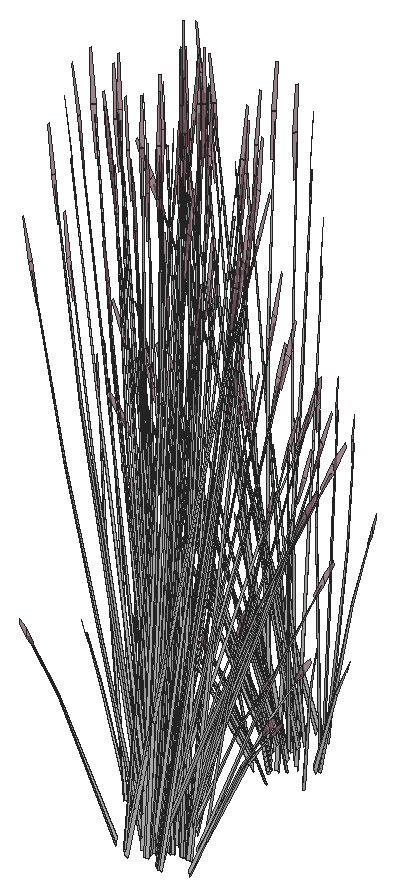
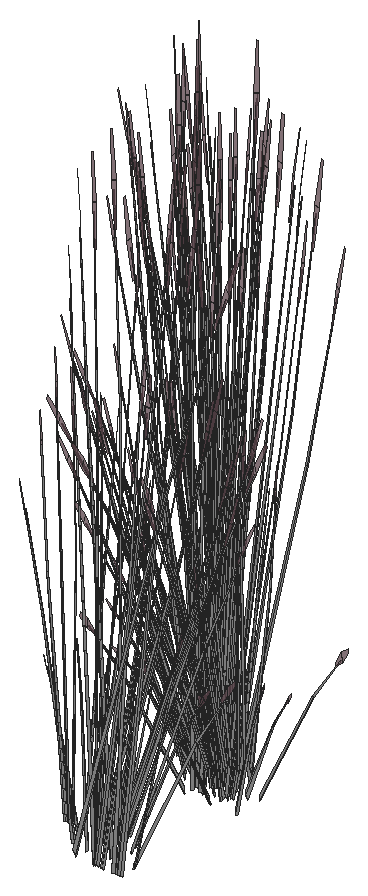
# SketchUp Ruby script. Lengths in inches.
U = 1.inch
M = Sketchup.active_model
def pt(a) = Geom::Point3d.new(a.map { |v| v * U })
def face(e, loops, mat)
  f = e.add_face(loops[0].map { |a| pt(a) })
  loops[1..].each { |l| e.add_face(l.map { |a| pt(a) }).erase! }
  f.material = f.back_material = mat if mat
  f
end
# faces: each face lists its corners as indices into pts; further lists are holes
def faces(e, pts, list, mat = nil) = list.each { |f| face(e, (f[0].is_a?(Array) ? f : [f]).map { |l| l.map { |i| pts[i] } }, mat) }
# xy, xz, yz: faces in a plane at the given z, y or x. An outline is a flat list of corners, or four numbers for a rectangle; further outlines are holes
def ring(l) = l.size == 4 ? [[l[0], l[1]], [l[2], l[1]], [l[2], l[3]], [l[0], l[3]]] : l.each_slice(2).to_a
def flat(e, list, mat, &to3) = list.each { |f| face(e, (f[0].is_a?(Array) ? f : [f]).map { |l| ring(l).map { |u, v| to3.(u, v) } }, mat) }
def xy(e, z, list, mat = nil) = flat(e, list, mat) { |x, y| [x, y, z] }
def xz(e, y, list, mat = nil) = flat(e, list, mat) { |x, z| [x, y, z] }
def yz(e, x, list, mat = nil) = flat(e, list, mat) { |y, z| [x, y, z] }
def lines(e, pts, list) = list.each { |a, b| e.add_line(pt(pts[a]), pt(pts[b])) }
# prism: a flat outline (further loops are holes) pulled along v
def prism(e, loops, v, mat = nil)
  f = face(e, loops, mat); d = Geom::Vector3d.new(v.map { |x| x * U })
  f.pushpull(f.normal.samedirection?(d) ? d.length : -d.length)
end
def box(e, o, s, mat = nil) = prism(e, [[o, [o[0] + s[0], o[1], o[2]], [o[0] + s[0], o[1] + s[1], o[2]], [o[0], o[1] + s[1], o[2]]]], [0, 0, s[2]], mat)
def at(x, y, z, deg = 0) = Geom::Transformation.translation(pt([x, y, z])) * Geom::Transformation.rotation(ORIGIN, Z_AXIS, deg.degrees)
def axes(o, x, y, z) = Geom::Transformation.new([*x, 0, *y, 0, *z, 0, *pt(o).to_a, 1])
def part(name) = M.definitions.add(name)
# library, detail: a bought-in or finely detailed component or shape, given as its bounding box
def library(name, o, s) = part(name).tap { |d| box(d.entities, o, s) }
def detail(e, o, s) = box(e.add_group.entities, o, s)
def put(e, d, t, mat = nil) = e.add_instance(d, t).tap { |i| i.material = mat if mat }
def group(e, t, mat = nil) = e.add_group.tap { |g| g.transformation = t; g.material = mat if mat }.entities
root = M.entities
M.materials.add("LightPink_Translucent").color = [144, 107, 117]
M.materials["LightPink_Translucent"].alpha = 0.75
M.materials.add("[_0053_Ivory_]").color = [200, 200, 200]
c1 = part("blade")
p = [[2.15,0.21,22],[0,0.17,0],[0.09,0.45,0],[2.18,0.31,22],[2.29,0.31,22],[0.38,0.45,0],
  [2.48,0.24,33],[2.49,0.24,33],[2.48,0.22,33]]
faces(c1.entities,p,[[0,1,2,3],[4,5,2,3],[6,3,4,7],[8,0,3,6]])
c2 = part("seeds")
p = [[0.3,-0.1,1.38],[-0.01,-0.03,1.59],[-0.01,-0.03,0.03],[0.14,-0.07,-0.07],[0.29,-0.03,3],[0.15,0.01,3.11]]
faces(c2.entities,p,[[0,1,2,3],[1,0,4,5]],"LightPink_Translucent")
c3 = part("blade with seeds")
put(c3.entities,c1,at(0,0,0))
put(c3.entities,c2,axes([2.4,0.25,30.99],[1.5799,-0.05474,1.17369],[-0.12525,1.92788,0.29478],[-0.07173,-0.02425,1.56792]))
put(root,c3,axes([642.95,172.91,128.71],[-0.63179,-0.1031,-0.62353],[0.13332,-0.63596,-0.16365],[-0.18854,-0.07706,1.37633]),"[_0053_Ivory_]")
put(root,c3,axes([643.95,171.57,129.01],[-0.50358,0.57069,0.45755],[-0.59827,-0.50377,0.17955],[0.1214,-0.05695,1.58856]),"[_0053_Ivory_]")
put(root,c3,axes([644.5,172.59,128.95],[-0.56493,-0.54126,-0.06131],[0.56528,-0.54159,0],[-0.01973,-0.0189,1.75571]),"[_0053_Ivory_]")
put(root,c3,axes([643.07,170.63,129.13],[-0.17545,0.62497,0.17642],[-0.64204,-0.17686,0.35086],[0.11091,-0.00304,1.60407]),"[_0053_Ivory_]")
put(root,c3,axes([642.81,171.13,128.25],[-0.59782,0.25177,1.28929],[-0.19028,-0.72239,0.50096],[0.36709,0.01202,1.46642]),"[_0053_Ivory_]")
put(root,c3,axes([644.41,171.32,129.27],[0.11717,-0.56122,0.1448],[0.57245,0.09742,-0.41347],[0.10418,0.05763,1.26744]),"[_0053_Ivory_]")
put(root,c3,axes([643.42,172.66,129.01],[0.76764,0.13249,0.45755],[-0.15622,0.74829,0.17955],[-0.11218,-0.07226,1.58856]),"[_0053_Ivory_]")
put(root,c3,axes([647.48,172.11,128.15],[-0.03174,-0.09547,1.76342],[0.22015,-0.55846,-0.26939],[0.22208,-0.00803,0.30037]),"[_0053_Ivory_]")
put(root,c3,axes([640.92,172.02,128.15],[0.0154,0.09911,1.76342],[-0.31051,0.51756,-0.26939],[-0.22056,-0.02609,0.30037]),"[_0053_Ivory_]")
put(root,c3,axes([644.17,171.47,129.37],[-0.36485,-0.52782,0.44739],[0.55265,-0.37168,-0.21531],[0.11807,0.06531,1.43643]),"[_0053_Ivory_]")
put(root,c3,axes([642.28,173.88,128.68],[-0.14267,-0.54795,-0.30978],[0.56663,-0.1556,0.30978],[-0.11423,-0.06319,1.38974]),"[_0053_Ivory_]")
put(root,c3,axes([643.01,173.85,129.13],[0.65264,-0.16691,0.17642],[0.16115,0.62115,0.35086],[-0.05821,-0.0905,1.60407]),"[_0053_Ivory_]")
put(root,c3,axes([644.35,171.5,129.32],[0.61322,-0.4175,-0.29095],[0.40778,0.58992,-0.50002],[0.1513,0.05991,1.59708]),"[_0053_Ivory_]")
put(root,c3,axes([646.79,172.61,131.18],[0.50475,0.17543,-0.35414],[-0.14722,0.5118,0.4572],[0.20322,-0.04693,0.87481]),"[_0053_Ivory_]")
put(root,c3,axes([642.125,174.12,128.67],[-0.56842,-0.31443,-0.49651],[0.33976,-0.56381,0],[-0.12946,-0.07161,1.57504]),"[_0053_Ivory_]")
put(root,c3,axes([645.9,170.39,128.67],[0.56842,0.31443,-0.49651],[-0.33976,0.56381,0],[0.12946,0.07161,1.57504]),"[_0053_Ivory_]")
put(root,c3,axes([644.82,172.1875,128.86],[0.67951,0,0],[0,0.65103,0],[0,0,1.78407]),"[_0053_Ivory_]")
put(root,c3,axes([643.67,173.01,129.32],[-0.61322,0.4175,-0.29095],[-0.40778,-0.58992,-0.50002],[-0.1513,-0.05991,1.59708]),"[_0053_Ivory_]")
put(root,c3,axes([645.01,170.66,129.13],[-0.65264,0.16691,0.17642],[-0.16115,-0.62115,0.35086],[0.05821,0.0905,1.60407]),"[_0053_Ivory_]")
put(root,c3,axes([645.42,171.97,130.53],[-0.25192,0.01424,1.71376],[0.16712,-0.61729,0.13857],[0.35901,0.03818,0.73262]),"[_0053_Ivory_]")
put(root,c3,axes([645.74,170.63,128.68],[0.14267,0.54795,-0.30978],[-0.56663,0.1556,0.30978],[0.11423,0.06319,1.38974]),"[_0053_Ivory_]")
put(root,c3,axes([644.6,171.86,129.03],[-0.76764,-0.13249,0.49198],[0.15622,-0.74829,0.19306],[0.11218,0.07226,1.70813]),"[_0053_Ivory_]")
put(root,c3,axes([643.99,173.7,128.86],[-0.19817,-0.54216,0],[0.56587,-0.18986,0],[0,0,1.54371]),"[_0053_Ivory_]")
put(root,c3,axes([643.61,173.19,129.27],[-0.11717,0.56122,0.1448],[-0.57245,-0.09742,-0.41347],[-0.10418,-0.05763,1.26744]),"[_0053_Ivory_]")
put(root,c3,axes([644.73,173.63,128.84],[0.63764,-0.21337,-0.19198],[0.22406,0.61462,0.00008],[0.07038,-0.02358,1.73897]),"[_0053_Ivory_]")
put(root,c3,axes([644.95,173.88,129.13],[0.17545,-0.62497,0.17642],[0.64204,0.17686,0.35086],[-0.11091,0.00304,1.60407]),"[_0053_Ivory_]")
put(root,c3,axes([644.81,172.47,128.87],[0.42396,0.40619,0],[-0.42396,0.40619,0],[0,0,1.69266]),"[_0053_Ivory_]")
put(root,c3,axes([645.95,172.29,129.13],[-0.47719,-0.45806,0.17642],[0.48088,-0.44429,0.35086],[-0.0527,0.09355,1.60407]),"[_0053_Ivory_]")
put(root,c3,axes([645.07,171.6,128.71],[0.63179,0.1031,-0.62353],[-0.13332,0.63596,-0.16365],[0.18854,0.07706,1.37633]),"[_0053_Ivory_]")
put(root,c3,axes([647.86,172.71,129.42],[-0.37526,0.10382,1.1486],[0.17664,-0.42906,0.84392],[0.19907,0.02936,0.25299]),"[_0053_Ivory_]")
put(root,c3,axes([643.85,173.95,128.85],[-0.61229,-0.28233,0],[0.29468,-0.58663,0],[0,0,1.62707]),"[_0053_Ivory_]")
put(root,c3,axes([644.36,173.2,129.12],[-0.59306,-0.50614,-0.25192],[0.49904,-0.56836,0.5513],[-0.1597,0.05921,1.68216]),"[_0053_Ivory_]")
put(root,c3,axes([642.8,174.17,129.13],[0.56842,0.31443,0.49651],[-0.33976,0.56381,0],[-0.12946,-0.07161,1.57504]),"[_0053_Ivory_]")
put(root,c3,axes([644.8,171.99,129.37],[0.29468,-0.56664,0.44739],[0.61229,0.27271,-0.21531],[0,0.13062,1.43643]),"[_0053_Ivory_]")
put(root,c3,axes([644.6875,172.32,128.95],[0,0.72727,-0.05637],[-0.75945,0,0],[0,0.02286,1.79368]),"[_0053_Ivory_]")
put(root,c3,axes([644.74,171.8,128.86],[0.36485,0.52782,-0.44739],[-0.55265,0.37168,0.21531],[0.11807,0.06531,1.43643]),"[_0053_Ivory_]")
put(root,c3,axes([647.21,174.03,130.58],[-0.11624,-0.52862,-0.03492],[0.54943,-0.12153,-0.15832],[0.11473,0.03351,0.52218]),"[_0053_Ivory_]")
put(root,c3,axes([642.47,174.5,129.03],[-0.37973,0.63014,0],[-0.6353,-0.35142,-0.51607],[-0.14469,-0.08004,1.63711]),"[_0053_Ivory_]")
put(root,c3,axes([646.35,172.31,129.13],[0,-0.62885,0.49651],[0.67951,0,0],[0,0.14322,1.57504]),"[_0053_Ivory_]")
put(root,c3,axes([644.65,172.78,129.37],[0.65953,-0.03882,0.44739],[0.05964,0.64439,-0.21531],[-0.11807,0.06531,1.43643]),"[_0053_Ivory_]")
put(root,c3,axes([645.06,172.12,129.27],[0.56587,-0.18339,0.1448],[0.19817,0.52368,-0.41347],[0,0.11525,1.26744]),"[_0053_Ivory_]")
put(root,c3,axes([644.06,173.09,128.86],[-0.65953,0.03882,-0.44739],[-0.05964,-0.64439,0.21531],[-0.11807,0.06531,1.43643]),"[_0053_Ivory_]")
put(root,c3,axes([647.16,173.4,129.24],[-0.14627,-0.15466,1.43002],[0.19032,-0.51164,-0.30754],[0.29594,0.06931,0.61141]),"[_0053_Ivory_]")
put(root,c3,axes([644.55,173.96,128.86],[0.61229,0.28233,0],[-0.29468,0.58663,0],[0,0,1.74954]),"[_0053_Ivory_]")
put(root,c3,axes([644.79,174.59,128.85],[-0.37499,-0.63235,-0.05142],[0.6353,-0.35142,0.51607],[-0.15655,0.0602,1.6363]),"[_0053_Ivory_]")
put(root,c3,axes([644.66,173.06,129.27],[0.44871,0.37783,0.1448],[-0.37428,0.42627,-0.41347],[-0.10418,0.05763,1.26744]),"[_0053_Ivory_]")
put(root,c3,axes([645.82,173.71,131.63],[0.60713,0.01514,-0.71045],[-0.04078,0.63759,0.08574],[0.25721,0.06729,1.00501]),"[_0053_Ivory_]")
put(root,c3,axes([645.13,174.22,129.13],[0.56842,-0.31443,0.49651],[0.33976,0.56381,0],[-0.12946,0.07161,1.57504]),"[_0053_Ivory_]")
put(root,c3,axes([644.32,173.72,128.94],[0.26406,0.72244,-0.06012],[-0.7545,0.25315,0],[0.00922,0.02523,1.72173]),"[_0053_Ivory_]")
put(root,c3,axes([644.62,174.51,128.68],[-0.56663,-0.1556,-0.30978],[0.14267,-0.54795,0.30978],[-0.11423,0.06319,1.38974]),"[_0053_Ivory_]")
put(root,c3,axes([646.81,172.42,129.03],[0.75945,0,0],[0,0.70283,-0.51607],[0,0.16007,1.63711]),"[_0053_Ivory_]")
put(root,c3,axes([646.51,172.78,128.85],[-0.75908,-0.00503,-0.04976],[0,-0.70283,0.49943],[-0.02386,0.16,1.58352]),"[_0053_Ivory_]")
put(root,c3,axes([644.86,172.16,129.32],[0.68399,0.30005,-0.29095],[-0.32934,0.63331,-0.50002],[0.0215,0.15549,1.59708]),"[_0053_Ivory_]")
put(root,c3,axes([640.09,174.5,129.42],[0.25312,-0.28501,1.1486],[0.09988,0.45119,0.84392],[-0.18292,0.08079,0.25299]),"[_0053_Ivory_]")
put(root,c3,axes([646.18,173.97,131.18],[0.34557,0.39372,-0.35414],[-0.39459,0.37271,0.4572],[0.20048,0.05671,0.87481]),"[_0053_Ivory_]")
put(root,c3,axes([646.35,172.88,128.68],[-0.42396,0.39235,-0.30978],[-0.42396,-0.39235,0.30978],[0,0.12637,1.38974]),"[_0053_Ivory_]")
put(root,c3,axes([644.52,172.92,129.32],[0.07077,0.71755,-0.29095],[-0.73712,0.04339,-0.50002],[-0.1298,0.09558,1.59708]),"[_0053_Ivory_]")
put(root,c3,axes([644.79,172.64,128.86],[-0.29468,0.56664,-0.44739],[-0.61229,-0.27271,0.21531],[0,0.13062,1.43643]),"[_0053_Ivory_]")
put(root,c3,axes([641.04,173.27,131.18],[-0.52868,0.08987,-0.35414],[-0.1396,-0.51376,0.4572],[-0.1515,0.13799,0.87481]),"[_0053_Ivory_]")
put(root,c3,axes([644.08,173.46,128.71],[-0.40909,0.47266,-0.62353],[-0.50819,-0.4286,-0.16365],[-0.16393,0.11791,1.37633]),"[_0053_Ivory_]")
put(root,c3,axes([644.81,174.26,128.98],[0.76036,0.2044,0.30756],[-0.19023,0.7306,-0.36492],[-0.12585,0.09144,1.64885]),"[_0053_Ivory_]")
put(root,c3,axes([644.75,174.75,128.67],[-0.56842,0.31443,-0.49651],[-0.33976,-0.56381,0],[-0.12946,0.07161,1.57504]),"[_0053_Ivory_]")
put(root,c3,axes([646.64,172.89,128.67],[0,0.62885,-0.49651],[-0.67951,0,0],[0,0.14322,1.57504]),"[_0053_Ivory_]")
put(root,c3,axes([644.94,172.96,130.53],[-0.2256,-0.10835,1.71376],[0.46687,-0.45453,0.13857],[0.29098,0.20505,0.73262]),"[_0053_Ivory_]")
put(root,c3,axes([645.78,174.2,129.42],[-0.34197,-0.18082,1.1486],[0.44156,-0.18372,0.84392],[0.1191,0.15563,0.25299]),"[_0053_Ivory_]")
put(root,c3,axes([641.96,172.76,130.53],[0.1517,-0.19322,1.71376],[0.38303,0.52154,0.13857],[-0.26271,0.23751,0.73262]),"[_0053_Ivory_]")
put(root,c3,axes([641.48,173.33,131.33],[0.15602,0.5742,-0.51099],[-0.59087,0.10045,-0.3958],[-0.16933,0.15423,0.97773]),"[_0053_Ivory_]")
put(root,c3,axes([645.27,174.66,129.03],[0.37973,0.63014,0],[-0.6353,0.35142,-0.51607],[-0.14469,0.08004,1.63711]),"[_0053_Ivory_]")
put(root,c3,axes([645.87,174.87,128.15],[0.04425,-0.09079,1.76342],[0.55709,-0.26738,-0.26939],[0.16889,0.13839,0.30037]),"[_0053_Ivory_]")
put(root,c3,axes([644.94,172.16,129.5],[-0.01659,-0.59209,1.41272],[0.75089,0.15348,0.59816],[-0.1776,0.32398,1.3335]),"[_0053_Ivory_]")
put(root,c3,axes([645.14,172.81,128.75],[0.2227,0.57576,-0.69212],[-0.64151,0.20736,-0.18165],[0.02462,0.19497,1.52773]),"[_0053_Ivory_]")
put(root,c3,axes([640.76,174.79,128.15],[0.08147,0.06283,1.76342],[0.13814,0.58211,-0.26939],[-0.18056,0.12413,0.30037]),"[_0053_Ivory_]")
put(root,c3,axes([645,174.45,131.33],[0.59932,-0.14948,-0.51099],[0.10484,0.56611,-0.3958],[0.16097,0.16223,0.97773]),"[_0053_Ivory_]")
put(root,c3,axes([645.83,175.02,129.32],[-0.38947,-0.01972,1.0506],[0.25721,-0.41888,0.58006],[0.15386,0.14882,0.8241]),"[_0053_Ivory_]")
put(root,c3,axes([641.84,173.24,130.53],[0.11309,-0.21615,1.71376],[0.47441,0.44731,0.13857],[-0.21402,0.27879,0.73262]),"[_0053_Ivory_]")
put(root,c3,axes([644.56,174,129.24],[0.01072,-0.20846,1.43002],[0.51218,-0.23285,-0.30754],[0.15811,0.2495,0.61141]),"[_0053_Ivory_]")
put(root,c3,axes([641.97,174.46,131.18],[-0.41095,0.33109,-0.35414],[-0.38901,-0.37805,0.4572],[-0.05919,0.19208,0.87481]),"[_0053_Ivory_]")
put(root,c3,axes([642.24,175.74,129.42],[-0.01572,-0.37392,1.1486],[0.39276,0.26669,0.84392],[-0.07724,0.17822,0.25299]),"[_0053_Ivory_]")
put(root,c3,axes([643.27,174.85,128.15],[0.09829,-0.03422,1.76342],[0.59126,0.18834,-0.26939],[0.01729,0.21228,0.30037]),"[_0053_Ivory_]")
put(root,c3,axes([642.38,174.3,131.66],[0.43478,0.42253,-0.5672],[-0.45929,0.37004,-0.43934],[-0.06615,0.21468,1.08528]),"[_0053_Ivory_]")
put(root,c3,axes([641.91,174.93,129.48],[0.55175,-0.11136,0.06507],[0.12684,0.44864,-0.86304],[-0.03498,0.22711,0.7736]),"[_0053_Ivory_]")
put(root,c3,axes([643.67,174.71,131.33],[0.59704,0.15764,-0.51099],[-0.20464,0.54049,-0.3958],[0.05475,0.21761,0.97773]),"[_0053_Ivory_]")
put(root,c3,axes([644.01,173.59,130.53],[-0.13883,-0.2019,1.71376],[0.64153,-0.16998,0.13857],[0.14499,0.31697,0.73262]),"[_0053_Ivory_]")
put(root,c3,axes([643.4,175.04,131.18],[-0.1831,0.48359,-0.35414],[-0.53419,-0.14105,0.4572],[0.04898,0.1947,0.87481]),"[_0053_Ivory_]")
put(root,c3,axes([642.25,174.11,131.99],[-0.0158,0.58168,-0.7886],[-0.66548,-0.03907,0.09517],[-0.07023,0.24643,1.11556]),"[_0053_Ivory_]")
put(root,c3,axes([642.88,173.69,130.53],[-0.01487,-0.24136,1.71376],[0.64429,0.16012,0.13857],[-0.03985,0.34396,0.73262]),"[_0053_Ivory_]")
put(root,c3,axes([643.46,174.61,131.63],[0.28988,0.51132,-0.71045],[-0.59671,0.28496,0.08574],[0.06778,0.24706,1.00501]),"[_0053_Ivory_]")
put(root,c3,axes([641.78,175.41,129.24],[0.19166,-0.0992,1.43002],[0.4732,0.29912,-0.30754],[-0.14084,0.25882,0.61141]),"[_0053_Ivory_]")
put(root,c3,axes([642.03,174.92,130.02],[0.01334,-0.32463,1.54345],[0.60018,0.17147,0.21329],[-0.052,0.34598,0.72882]),"[_0053_Ivory_]")
put(root,c3,axes([642.49,186.4,130.53],[0.13883,0.2019,1.71376],[-0.64153,0.16998,0.13857],[-0.14499,-0.31697,0.73262]),"[_0053_Ivory_]")
put(root,c3,axes([644.98,186.11,129.24],[-0.17264,0.12729,1.43002],[-0.51703,-0.22279,-0.30754],[0.09584,-0.27707,0.61141]),"[_0053_Ivory_]")
put(root,c3,axes([644.2,186.55,131.63],[-0.28988,-0.51132,-0.71045],[0.59671,-0.28496,0.08574],[-0.06778,-0.24706,1.00501]),"[_0053_Ivory_]")
put(root,c3,axes([642.3125,185.87,129.24],[-0.03678,0.20572,1.43002],[-0.53767,0.17221,-0.30754],[-0.12568,-0.26589,0.61141]),"[_0053_Ivory_]")
put(root,c3,axes([643.7,185.42,128.15],[-0.10187,0.02266,1.76342],[-0.56336,-0.25503,-0.26939],[0.00945,-0.21273,0.30037]),"[_0053_Ivory_]")
put(root,c3,axes([645.4,187.05,131.63],[0.0158,-0.58168,-0.71045],[0.66548,0.03907,0.08574],[0.07023,-0.24643,1.00501]),"[_0053_Ivory_]")
put(root,c3,axes([644.25,186.12,131.18],[0.1831,-0.48359,-0.35414],[0.53419,0.14105,0.4572],[-0.04898,-0.1947,0.87481]),"[_0053_Ivory_]")
put(root,c3,axes([644.65,186.75,130.53],[-0.11309,0.21615,1.71376],[-0.47441,-0.44731,0.13857],[0.21402,-0.27879,0.73262]),"[_0053_Ivory_]")
put(root,c3,axes([643.98,186.45,131.33],[-0.59704,-0.15764,-0.51099],[0.20464,-0.54049,-0.3958],[-0.05475,-0.21761,0.97773]),"[_0053_Ivory_]")
put(root,c3,axes([644.35,185.09,129.42],[0.07791,0.3667,1.1486],[-0.43222,-0.2031,0.84392],[0.04651,-0.18776,0.25299]),"[_0053_Ivory_]")
put(root,c3,axes([645.27,186.86,131.33],[-0.43478,-0.42253,-0.51099],[0.45929,-0.37004,-0.3958],[0.06615,-0.21468,0.97773]),"[_0053_Ivory_]")
put(root,c3,axes([645.68,186.7,131.18],[0.41095,-0.33109,-0.35414],[0.38901,0.37805,0.4572],[0.05919,-0.19208,0.87481]),"[_0053_Ivory_]")
put(root,c3,axes([642.125,185.53,129.42],[0.31682,0.21887,1.1486],[-0.4614,0.13157,0.84392],[-0.09872,-0.16821,0.25299]),"[_0053_Ivory_]")
put(root,c3,axes([642.89,186.69,131.63],[-0.51789,-0.30395,-0.71045],[0.36805,-0.53263,0.08574],[-0.18764,-0.18149,1.00501]),"[_0053_Ivory_]")
put(root,c3,axes([642.71,186.29,131.18],[-0.0938,-0.50652,-0.35414],[0.53623,-0.13375,0.4572],[-0.14403,-0.14515,0.87481]),"[_0053_Ivory_]")
put(root,c3,axes([641.875,186.19,128.15],[-0.05883,0.08284,1.76342],[-0.59454,0.17861,-0.26939],[-0.14363,-0.16248,0.30037]),"[_0053_Ivory_]")
put(root,c3,axes([642.86,188.47,128.75],[-0.24943,-0.64486,-0.69835],[0.71849,-0.23224,-0.18329],[-0.02757,-0.21836,1.54149]),"[_0053_Ivory_]")
put(root,c3,axes([646.19,186.5,128.15],[-0.0909,-0.04954,1.76342],[-0.2335,-0.55347,-0.26939],[0.15752,-0.1502,0.30037]),"[_0053_Ivory_]")
put(root,c3,axes([642.65,186.71,131.33],[-0.59932,0.14948,-0.51099],[-0.10484,-0.56611,-0.3958],[-0.16097,-0.16223,0.97773]),"[_0053_Ivory_]")
put(root,c3,axes([646.1875,188.0625,131.63],[0.31725,-0.49618,-0.71045],[0.55593,0.35263,0.08574],[0.18942,-0.17977,1.00501]),"[_0053_Ivory_]")
put(root,c3,axes([642.76,186.62,129.03],[-0.37973,-0.63014,0],[0.6353,-0.35142,-0.51607],[0.14469,-0.08004,1.63711]),"[_0053_Ivory_]")
put(root,c3,axes([646.17,187.83,131.33],[-0.15602,-0.5742,-0.51099],[0.59087,-0.10045,-0.3958],[0.16933,-0.15423,0.97773]),"[_0053_Ivory_]")
put(root,c3,axes([643.59,185.86,128.78],[-0.4197,0.36076,-0.03893],[-0.38456,-0.39511,-0.17649],[-0.02707,-0.11196,0.58215]),"[_0053_Ivory_]")
put(root,c3,axes([644.13,190.13,129.98],[0.52485,0.25358,1.51261],[-0.51417,0.54629,0.59816],[-0.23031,-0.32378,1.26806]),"[_0053_Ivory_]")
put(root,c3,axes([641.39,188.38,128.67],[0,-0.62885,-0.49651],[0.67951,0,0],[0,-0.14322,1.57504]),"[_0053_Ivory_]")
put(root,c3,axes([643.27,186.52,128.67],[0.56842,-0.31443,-0.49651],[0.33976,0.56381,0],[0.12946,-0.07161,1.57504]),"[_0053_Ivory_]")
put(root,c3,axes([646.65,187.6,129.24],[-0.21697,-0.01863,1.43002],[-0.22228,-0.49966,-0.30754],[0.26655,-0.14135,0.61141]),"[_0053_Ivory_]")
put(root,c3,axes([643.95,187.81,128.71],[0.40909,-0.47266,-0.62353],[0.50819,0.4286,-0.16365],[0.16393,-0.11791,1.37633]),"[_0053_Ivory_]")
put(root,c3,axes([646.9,186.6875,129.42],[-0.2023,0.32011,1.1486],[-0.17388,-0.43009,0.84392],[0.16708,-0.10777,0.25299]),"[_0053_Ivory_]")
put(root,c3,axes([646.61,187.89,131.18],[0.52868,-0.08987,-0.35414],[0.1396,0.51376,0.4572],[0.1515,-0.13799,0.87481]),"[_0053_Ivory_]")
put(root,c3,axes([643.24,188.64,128.86],[0.29468,-0.56664,-0.44739],[0.61229,0.27271,0.21531],[0,-0.13062,1.43643]),"[_0053_Ivory_]")
put(root,c3,axes([641.47,187.18,131.18],[-0.34557,-0.39372,-0.35414],[0.39459,-0.37271,0.4572],[-0.20048,-0.05671,0.87481]),"[_0053_Ivory_]")
put(root,c3,axes([643.5,188.36,129.32],[-0.07077,-0.71755,-0.29095],[0.73712,-0.04339,-0.50002],[0.1298,-0.09558,1.59708]),"[_0053_Ivory_]")
put(root,c3,axes([641.68,188.39,128.68],[0.42396,-0.39235,-0.30978],[0.42396,0.39235,0.30978],[0,-0.12637,1.38974]),"[_0053_Ivory_]")
put(root,c3,axes([641.51,186.51,128.78],[-0.1752,0.51349,-0.03893],[-0.53924,-0.15795,-0.17649],[-0.08187,-0.08399,0.58215]),"[_0053_Ivory_]")
put(root,c3,axes([643.16,189.11,129.32],[-0.68399,-0.30005,-0.29095],[0.32934,-0.63331,-0.50002],[-0.0215,-0.15549,1.59708]),"[_0053_Ivory_]")
put(root,c3,axes([641.22,188.86,129.03],[-0.75945,0,0],[0,-0.70283,-0.51607],[0,-0.16007,1.63711]),"[_0053_Ivory_]")
